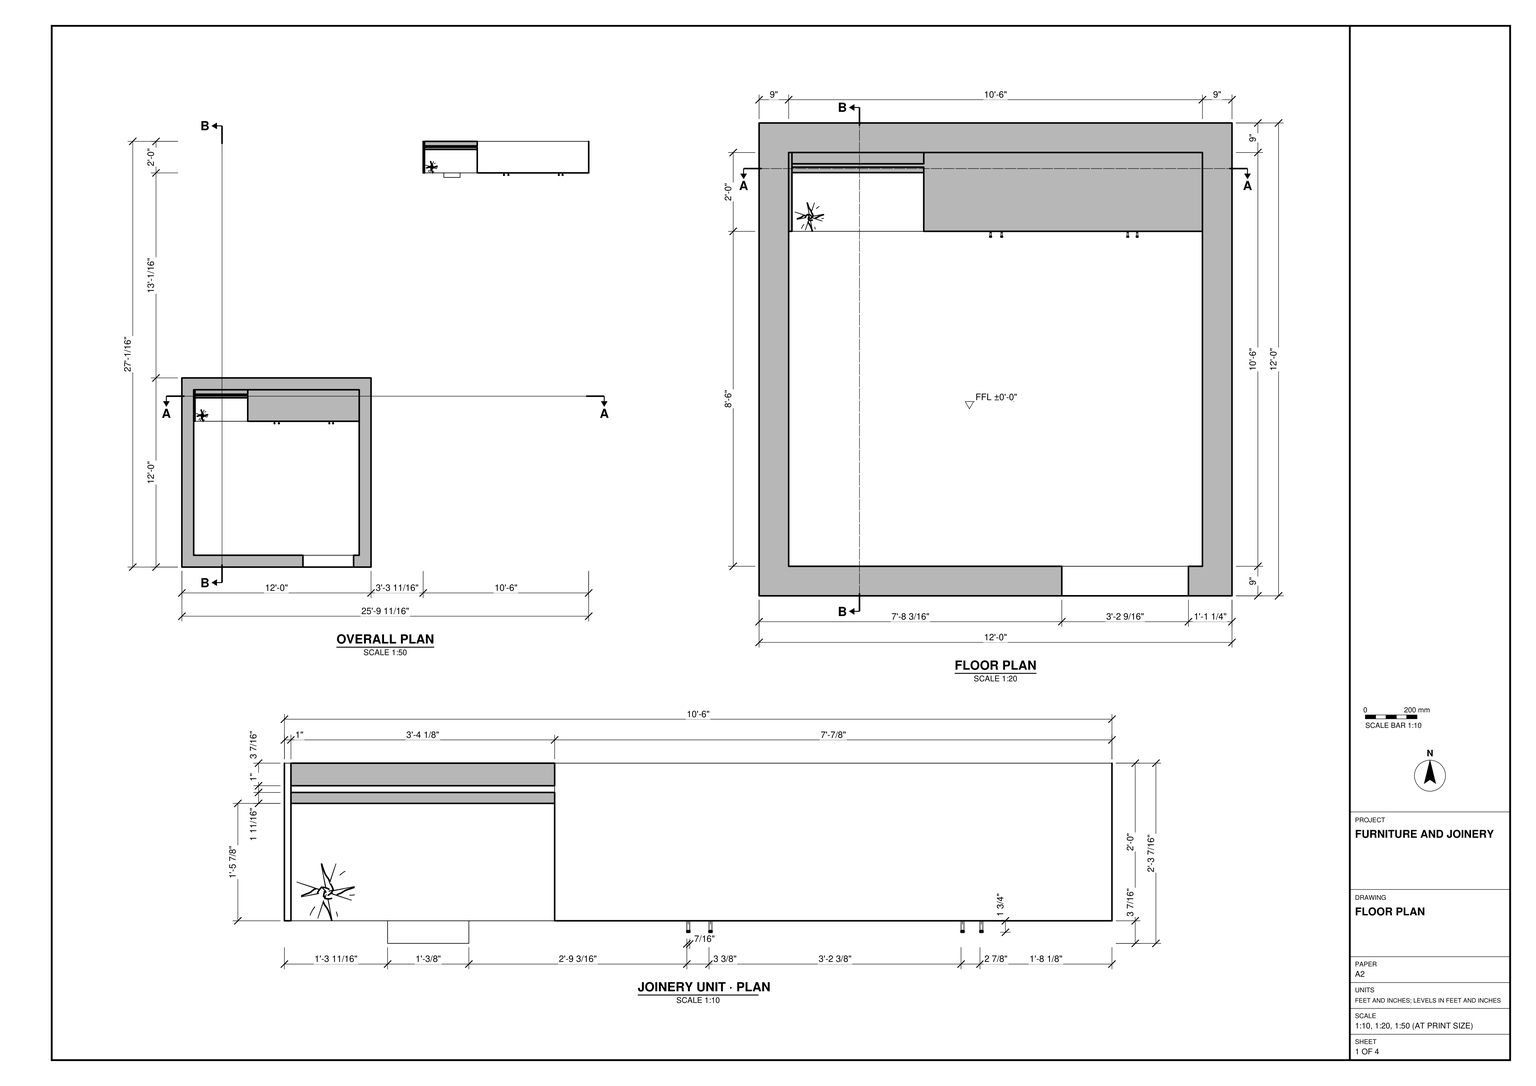
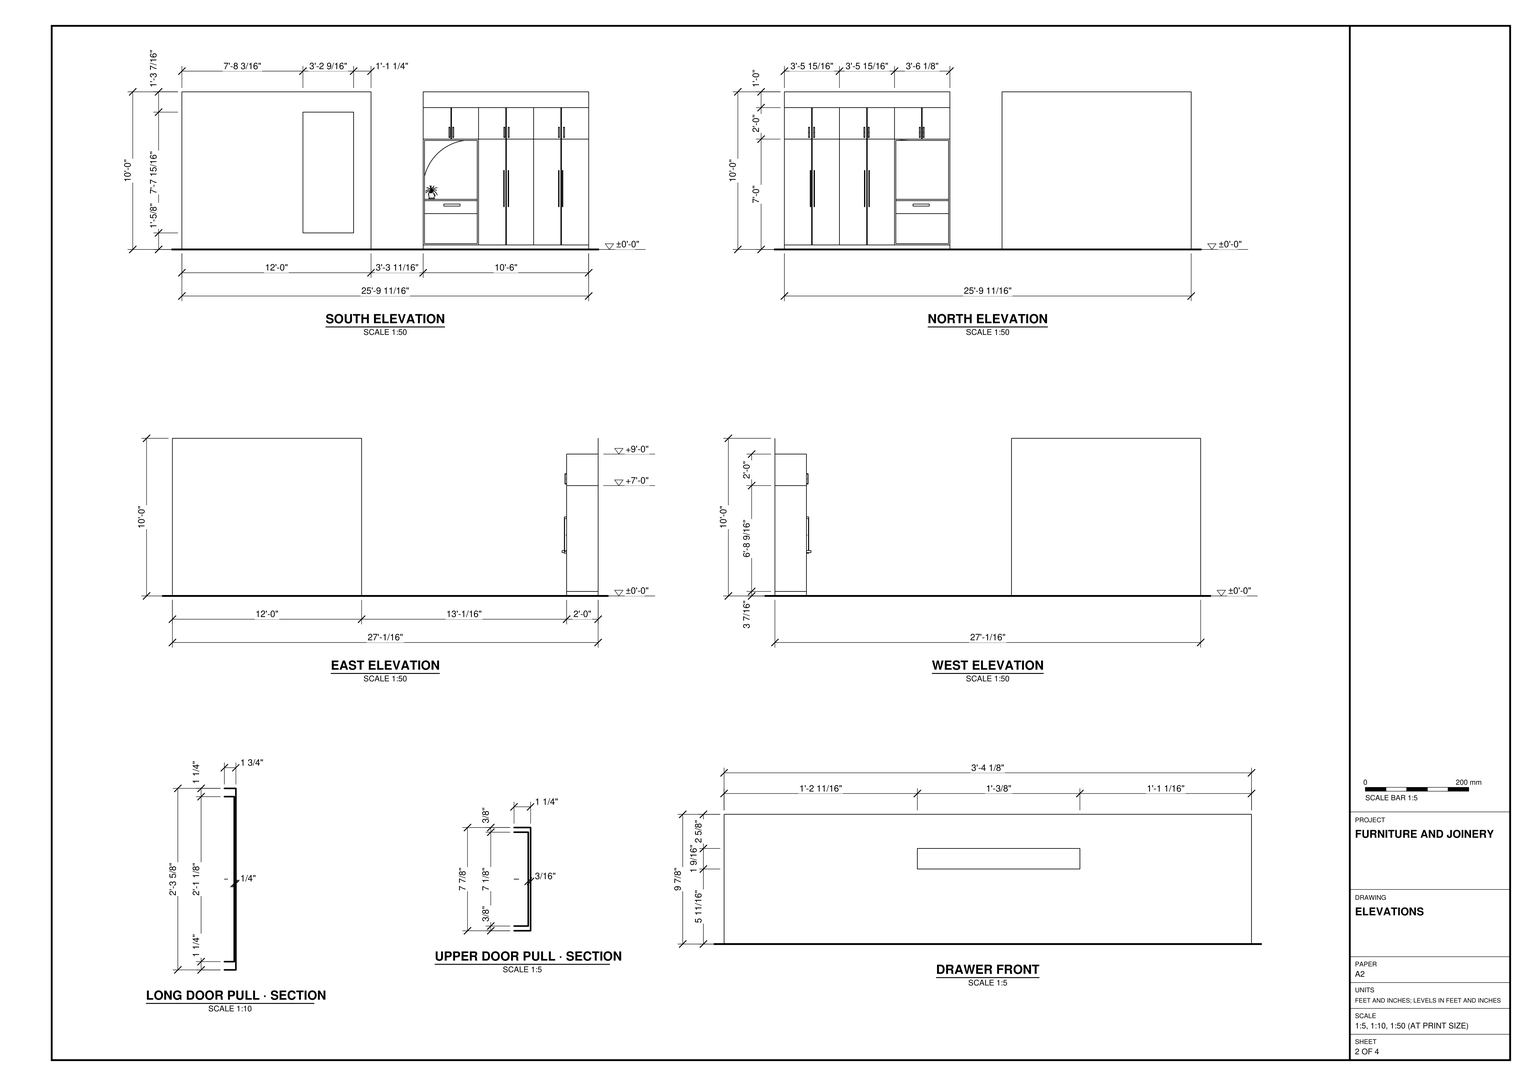
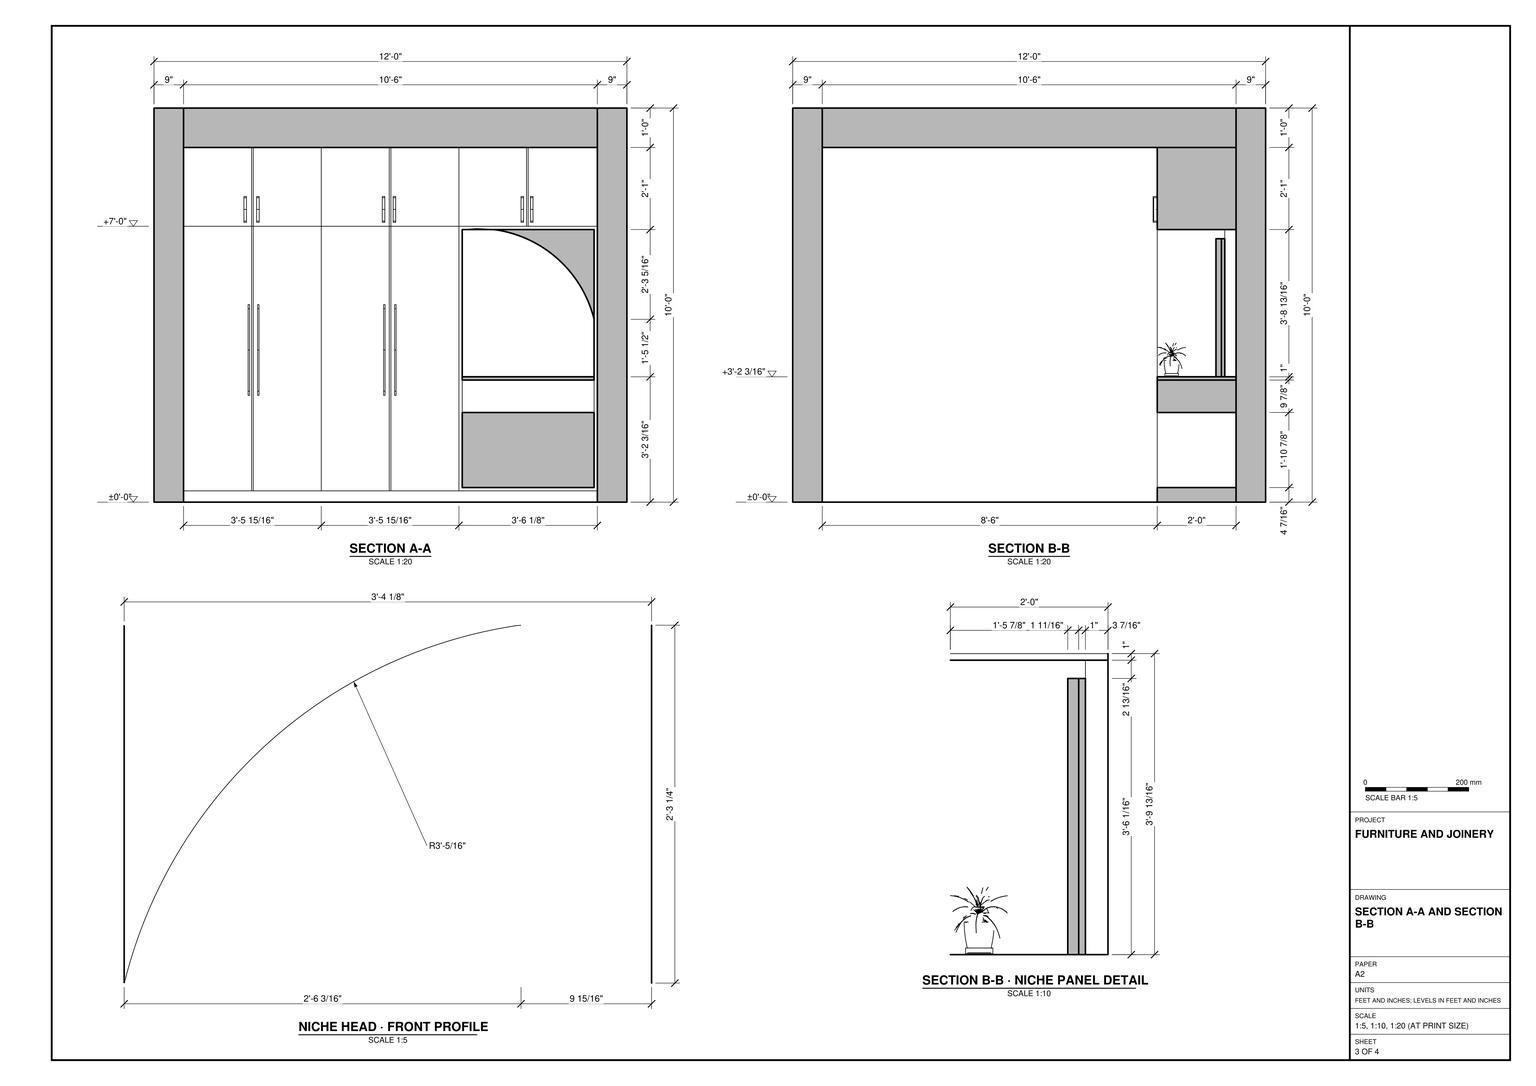
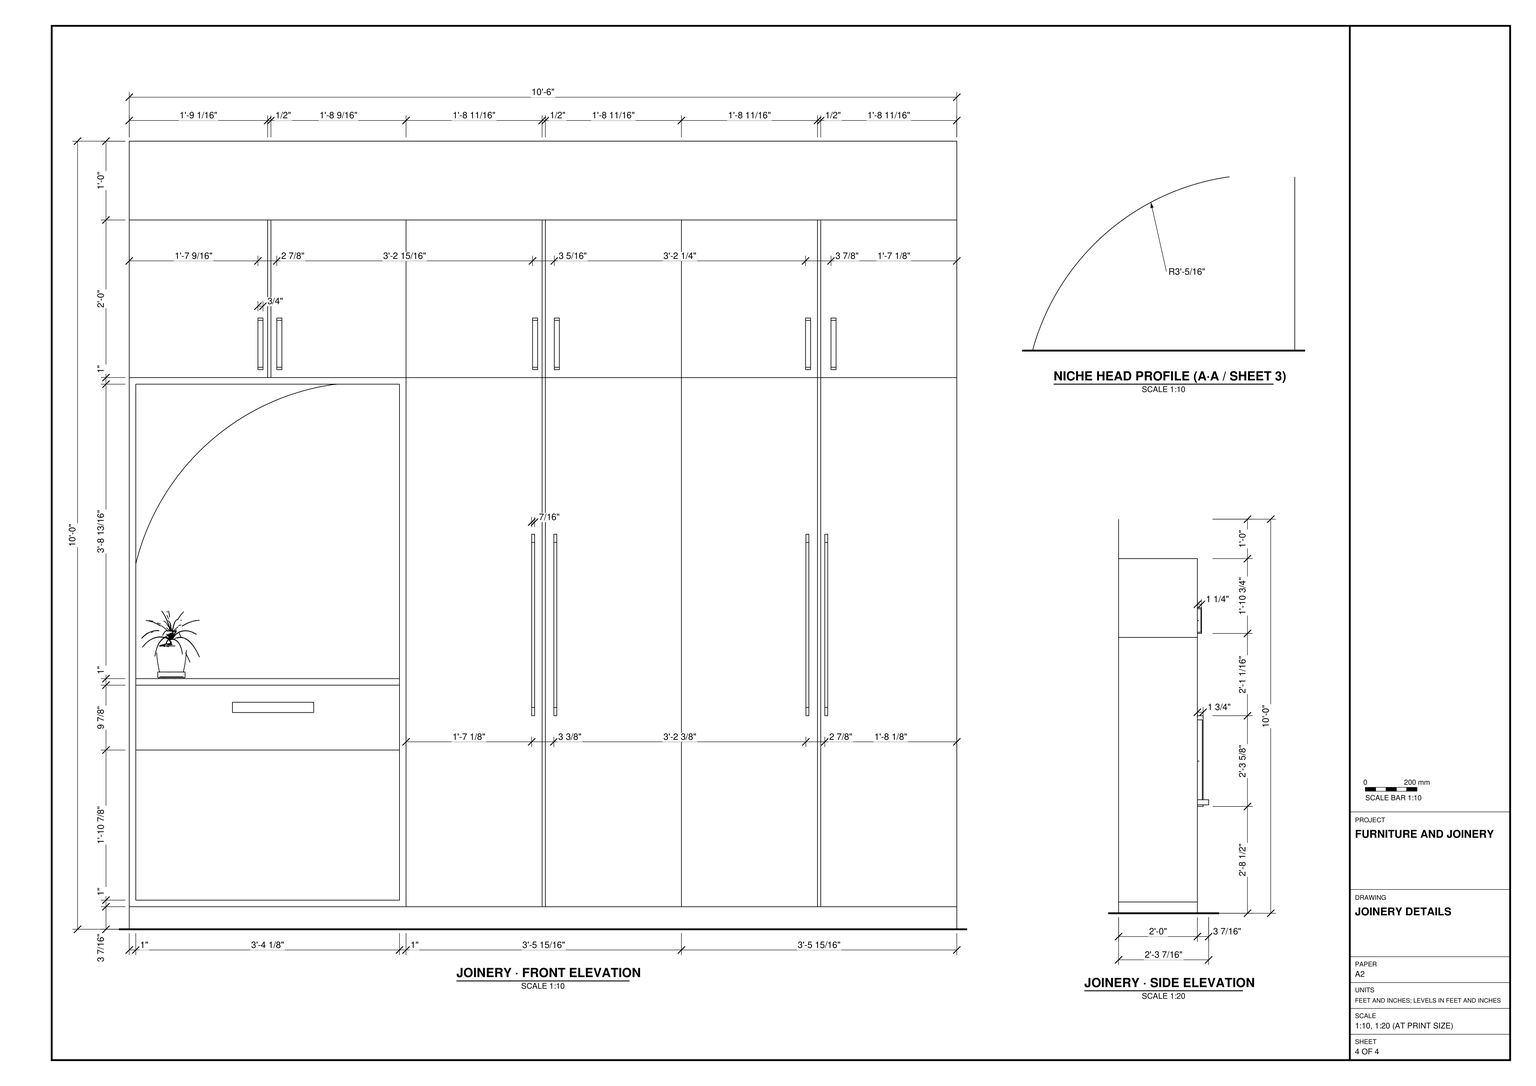
Work in feet and inches in SketchUp. Use task_files/diagram_01.pdf to model the wardrobe both in its room and as a separate unit. Follow the overall plan for their relative positions: the separate unit stands to the northeast of the room, with its long axis parallel to the fitted wardrobe. The complete layout measures 25'-9 11/16" along X, 27'-1/16" along Y and 10'-0" along Z. Use ±0'-0" as the finished floor level.

Build the 12'-0" square room with 9" walls, the top slab shown in section and the raised rectangular opening near the east end of the south wall. Fit the wardrobe across the north wall. Make its body 10'-6" wide and 2'-0" deep. Follow the elevations for the plinth, the paired tall doors and the continuous row of smaller cupboard doors above. Place the long pulls at the meeting edges of the tall doors and the shorter pulls on the upper doors.

At the end bay, model the shelf, drawer with horizontal pull, and upright niche panel. Use the front profile to shape the niche head: the curve rises from one side and flattens toward the top. Decor and loose items, including the plant on the niche shelf, may be any suitable library components. Keep the walls, slabs and each joinery piece in separate groups or components, and use components for repeated parts. Save one SketchUp model as output_files/fitted_wardrobe_with_a_curved_display_niche.skp.

# SketchUp Ruby script. Lengths in inches.
U = 1.inch
M = Sketchup.active_model
def pt(a) = Geom::Point3d.new(a.map { |v| v * U })
def face(e, loops, mat)
  f = e.add_face(loops[0].map { |a| pt(a) })
  loops[1..].each { |l| e.add_face(l.map { |a| pt(a) }).erase! }
  f.material = f.back_material = mat if mat
  f
end
# faces: each face lists its corners as indices into pts; further lists are holes
def faces(e, pts, list, mat = nil) = list.each { |f| face(e, (f[0].is_a?(Array) ? f : [f]).map { |l| l.map { |i| pts[i] } }, mat) }
# xy, xz, yz: faces in a plane at the given z, y or x. An outline is a flat list of corners, or four numbers for a rectangle; further outlines are holes
def ring(l) = l.size == 4 ? [[l[0], l[1]], [l[2], l[1]], [l[2], l[3]], [l[0], l[3]]] : l.each_slice(2).to_a
def flat(e, list, mat, &to3) = list.each { |f| face(e, (f[0].is_a?(Array) ? f : [f]).map { |l| ring(l).map { |u, v| to3.(u, v) } }, mat) }
def xy(e, z, list, mat = nil) = flat(e, list, mat) { |x, y| [x, y, z] }
def xz(e, y, list, mat = nil) = flat(e, list, mat) { |x, z| [x, y, z] }
def yz(e, x, list, mat = nil) = flat(e, list, mat) { |y, z| [x, y, z] }
def lines(e, pts, list) = list.each { |a, b| e.add_line(pt(pts[a]), pt(pts[b])) }
# prism: a flat outline (further loops are holes) pulled along v
def prism(e, loops, v, mat = nil)
  f = face(e, loops, mat); d = Geom::Vector3d.new(v.map { |x| x * U })
  f.pushpull(f.normal.samedirection?(d) ? d.length : -d.length)
end
def box(e, o, s, mat = nil) = prism(e, [[o, [o[0] + s[0], o[1], o[2]], [o[0] + s[0], o[1] + s[1], o[2]], [o[0], o[1] + s[1], o[2]]]], [0, 0, s[2]], mat)
def at(x, y, z, deg = 0) = Geom::Transformation.translation(pt([x, y, z])) * Geom::Transformation.rotation(ORIGIN, Z_AXIS, deg.degrees)
def axes(o, x, y, z) = Geom::Transformation.new([*x, 0, *y, 0, *z, 0, *pt(o).to_a, 1])
def part(name) = M.definitions.add(name)
# library, detail: a bought-in or finely detailed component or shape, given as its bounding box
def library(name, o, s) = part(name).tap { |d| box(d.entities, o, s) }
def detail(e, o, s) = box(e.add_group.entities, o, s)
def put(e, d, t, mat = nil) = e.add_instance(d, t).tap { |i| i.material = mat if mat }
def group(e, t, mat = nil) = e.add_group.tap { |g| g.transformation = t; g.material = mat if mat }.entities
root = M.entities
M.materials.add("[Color C05]").color = [255, 127, 0]
M.materials.add("[Color M09]").color = [0, 0, 0]
c1 = library("Fitted wardrobe",[0,-25.75,0],[126,25.75,120])
c2 = part("Component\#4")
xy(c2.entities,-12,[[[0,0,126,126],[24,24,102,102]],[[24,24,102,102],[36,36,90,90]],[37.84,37.84,88.16,88.16]])
xy(c2.entities,-12,[[[36,36,90,90],[37.84,37.84,88.16,88.16]]],"[Color C05]")
xy(c2.entities,0,[[0,0,126,126]])
xz(c2.entities,0,[[0,-12,126,0]])
xz(c2.entities,126,[[0,-12,126,0]])
yz(c2.entities,0,[[0,-12,126,0]])
yz(c2.entities,126,[[0,-12,126,0]])
xy(root,0,[[[0,0,144,144],[9,9,135,135]],[9,9,135,135]])
xy(root,12.6,[[92.17,0,130.73,9]])
xy(root,33.01,[[199.41,296.65,211.79,300.09]],"[Color M09]")
xy(root,34.57,[[199.41,296.65,211.79,300.09]],"[Color M09]")
xy(root,104.54,[[92.17,0,130.73,9]])
xy(root,120,[[[0,0,144,144],[9,9,135,135]]])
xz(root,0,[[[0,0,144,120],[92.17,12.6,130.73,104.54]],[92.17,12.6,130.73,104.54]])
xz(root,9,[[[9,0,135,120],[92.17,12.6,130.73,104.54]]])
xz(root,135,[[9,0,135,120]])
xz(root,144,[[0,0,144,120]])
xz(root,296.65,[[199.41,33.01,211.79,34.57]],"[Color M09]")
xz(root,300.09,[[199.41,33.01,211.79,34.57]])
yz(root,0,[[0,0,144,120]])
yz(root,9,[[9,0,135,120]])
yz(root,92.17,[[0,12.6,9,104.54]])
yz(root,130.73,[[0,12.6,9,104.54]])
yz(root,135,[[9,0,135,120]])
yz(root,144,[[0,0,144,120]])
yz(root,199.41,[[296.65,33.01,300.09,34.57]],"[Color M09]")
yz(root,211.79,[[296.65,33.01,300.09,34.57]],"[Color M09]")
put(root,c1,at(9,135,0))
put(root,c1,at(183.7,324.09,0))
put(root,c2,at(9,9,120))
